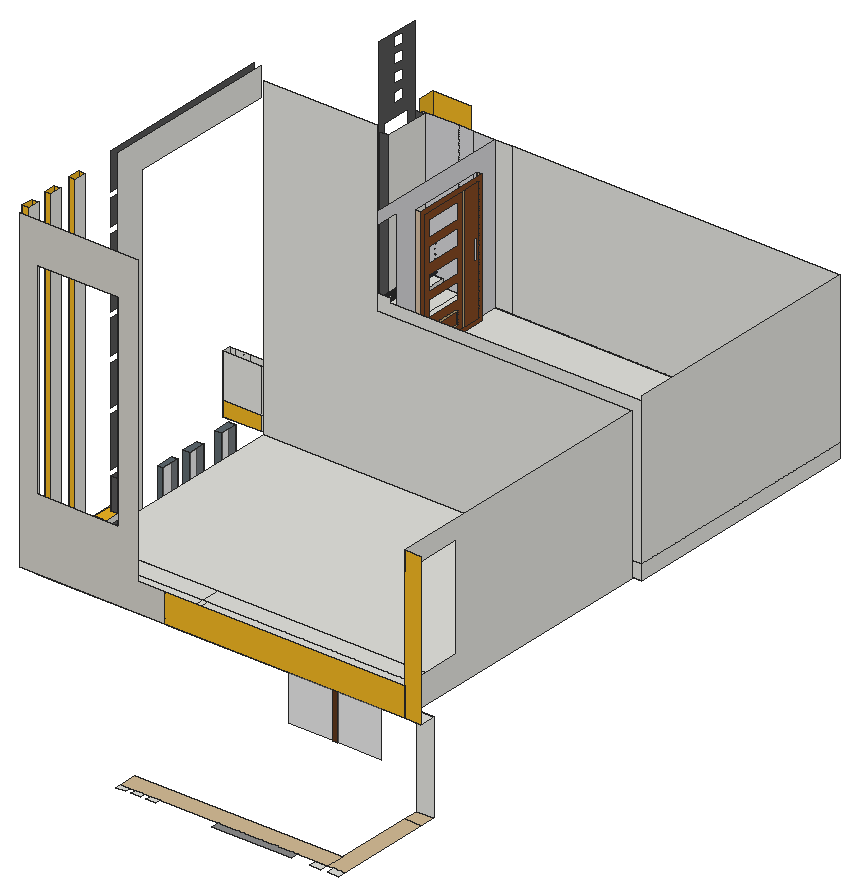
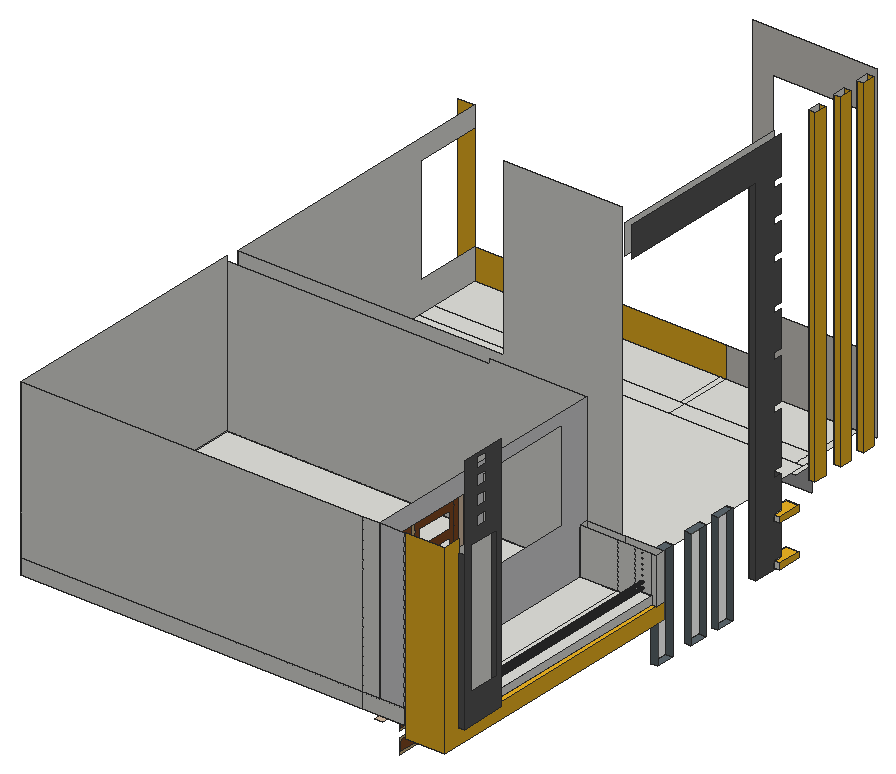
# SketchUp Ruby script. Lengths in inches.
U = 1.inch
M = Sketchup.active_model
def pt(a) = Geom::Point3d.new(a.map { |v| v * U })
def face(e, loops, mat)
  f = e.add_face(loops[0].map { |a| pt(a) })
  loops[1..].each { |l| e.add_face(l.map { |a| pt(a) }).erase! }
  f.material = f.back_material = mat if mat
  f
end
# faces: each face lists its corners as indices into pts; further lists are holes
def faces(e, pts, list, mat = nil) = list.each { |f| face(e, (f[0].is_a?(Array) ? f : [f]).map { |l| l.map { |i| pts[i] } }, mat) }
# xy, xz, yz: faces in a plane at the given z, y or x. An outline is a flat list of corners, or four numbers for a rectangle; further outlines are holes
def ring(l) = l.size == 4 ? [[l[0], l[1]], [l[2], l[1]], [l[2], l[3]], [l[0], l[3]]] : l.each_slice(2).to_a
def flat(e, list, mat, &to3) = list.each { |f| face(e, (f[0].is_a?(Array) ? f : [f]).map { |l| ring(l).map { |u, v| to3.(u, v) } }, mat) }
def xy(e, z, list, mat = nil) = flat(e, list, mat) { |x, y| [x, y, z] }
def xz(e, y, list, mat = nil) = flat(e, list, mat) { |x, z| [x, y, z] }
def yz(e, x, list, mat = nil) = flat(e, list, mat) { |y, z| [x, y, z] }
def lines(e, pts, list) = list.each { |a, b| e.add_line(pt(pts[a]), pt(pts[b])) }
# prism: a flat outline (further loops are holes) pulled along v
def prism(e, loops, v, mat = nil)
  f = face(e, loops, mat); d = Geom::Vector3d.new(v.map { |x| x * U })
  f.pushpull(f.normal.samedirection?(d) ? d.length : -d.length)
end
def box(e, o, s, mat = nil) = prism(e, [[o, [o[0] + s[0], o[1], o[2]], [o[0] + s[0], o[1] + s[1], o[2]], [o[0], o[1] + s[1], o[2]]]], [0, 0, s[2]], mat)
def at(x, y, z, deg = 0) = Geom::Transformation.translation(pt([x, y, z])) * Geom::Transformation.rotation(ORIGIN, Z_AXIS, deg.degrees)
def axes(o, x, y, z) = Geom::Transformation.new([*x, 0, *y, 0, *z, 0, *pt(o).to_a, 1])
def part(name) = M.definitions.add(name)
# library, detail: a bought-in or finely detailed component or shape, given as its bounding box
def library(name, o, s) = part(name).tap { |d| box(d.entities, o, s) }
def detail(e, o, s) = box(e.add_group.entities, o, s)
def put(e, d, t, mat = nil) = e.add_instance(d, t).tap { |i| i.material = mat if mat }
def group(e, t, mat = nil) = e.add_group.tap { |g| g.transformation = t; g.material = mat if mat }.entities
root = M.entities
M.materials.add("[0045_Goldenrod]").color = [239, 181, 35]
M.materials.add("[Blinds Vertical Pattern]").color = [212, 212, 214]
M.materials.add("[Color M04]").color = [142, 142, 142]
M.materials.add("[Color M06]").color = [86, 86, 86]
M.materials.add("[Color M07]").color = [58, 58, 58]
M.materials.add("[Fencing Picket Concave]").color = [160, 160, 160]
M.materials.add("[Formica Beige]").color = [211, 187, 149]
M.materials.add("[Formica Laminate Light]").color = [213, 189, 164]
M.materials.add("[Formica Speckled Grey]").color = [94, 105, 111]
M.materials.add("[Tile Travertine 2 inch]").color = [211, 208, 201]
M.materials.add("[Translucent Glass Gray]").color = [145, 145, 145]
M.materials["[Translucent Glass Gray]"].alpha = 0.5
M.materials.add("[Translucent Glass Gray]1").color = [128, 128, 128]
M.materials["[Translucent Glass Gray]1"].alpha = 0.5
M.materials.add("[Wood Cherry Original]").color = [130, 73, 35]
M.materials.add("[Wood Floor Light]").color = [204, 176, 127]
M.materials.add("[Wood Veneer 01]").color = [96, 56, 29]
xy(root,89.5625,[[499.38,0,512.5625,9.1875],[520.19,0,533.375,9.1875],[265.43,2.6875,276.6,9.1875],[283.37,2.6875,294.54,9.1875],[301.06,2.6875,312.23,9.1875]])
xy(root,89.5625,[[382.41,0,477.59,9.1875]],"[Color M04]")
xy(root,89.5625,[[265.43,9.1875,513.45,31.125],[513.45,9.1875,533.375,123.625],[513.45,123.625,533.375,142.4375]],"[Formica Beige]")
xy(root,101.04,[[53.375,329.87,59.9375,351.12],[53.375,367.37,61.125,388.62],[53.375,415.12,61.375,436.37]],"[Formica Speckled Grey]")
xy(root,134.2,[[45.3125,270.46,53.375,306.125]],"[Color M06]")
xy(root,136.59,[[38.625,253.03,38.625,280.03,45.3125,280.03,45.3125,270.46,53.375,270.46,53.375,253.03]],"[0045_Goldenrod]")
xy(root,143.41,[[38.625,253.03,53.375,253.03,53.375,270.46,45.3125,270.46,45.3125,280.03,38.625,280.03]],"[0045_Goldenrod]")
xy(root,160.59,[[116.75,663.47,125.57,751.59]],"[Formica Laminate Light]")
xy(root,164.17,[[106.94,539.02,116.75,631.05],[116.75,539.02,128.38,631.05]])
xy(root,167.75,[[311.03,171.21,433.4,181.59],[311.03,181.59,433.4,197.15]])
xy(root,174.66,[[106.94,528.53,116.75,641.54]])
xy(root,183.35,[[295.4375,171.21,449,181.59]])
xy(root,184.34,[[38.625,253.03,38.625,280.03,45.3125,280.03,45.3125,270.46,53.375,270.46,53.375,253.03]],"[0045_Goldenrod]")
xy(root,185.6875,[[53.375,483.625,116.75,779.875],[116.75,483.625,509.21,779.875]])
xy(root,185.6875,[[8.375,483.625,53.375,779.875],[8.375,779.875,18.625,797.6875]],"[0045_Goldenrod]")
xy(root,186,[[81.47,181.59,226.34,204.11]])
xy(root,191.16,[[38.625,253.03,53.375,253.03,53.375,270.46,45.3125,270.46,45.3125,280.03,38.625,280.03]],"[0045_Goldenrod]")
xy(root,198,[[73.3,123.625,81.47,181.59],[81.47,123.625,226.34,181.59],[226.34,123.625,231.56,181.59],[231.56,123.625,513.45,181.59],[513.45,123.625,533.375,142.4375],
  [73.3,181.59,81.47,204.11],[81.47,181.59,226.34,204.11],[226.34,181.59,513.45,204.11],[73.3,204.11,513.45,463.7]])
xy(root,198,[[45.75,136.75,53.375,151.32],[45.75,169.81,53.375,184.38],[45.75,206.12,53.375,220.7]],"[0045_Goldenrod]")
xy(root,203.25,[[8.375,483.625,97.02,493.85],[97.02,483.625,97.02,660.4,103.59,660.4,103.59,752.02,97.02,752.02,97.02,779.875,509.21,779.875,509.21,483.625],[14.37,493.85,33.87,779.875],[33.87,493.85,53.375,779.875],[53.375,493.85,97.02,493.85,97.02,660.4,103.59,660.4,103.59,752.02,97.02,752.02,97.02,779.875,53.375,779.875],
  [8.375,724.47,14.37,777.2],[8.375,777.2,14.37,779.875]])
xy(root,203.25,[[8.375,493.85,14.37,724.47]],"[0045_Goldenrod]")
xy(root,203.25,[[2.5625,724.47,8.375,777.2]],"[Color M06]")
xy(root,212.375,[[14.37,493.85,33.87,779.875]])
xy(root,216.42,[[53.375,329.87,59.9375,351.12],[53.375,367.37,61.125,388.62],[53.375,415.12,61.375,436.37]],"[Formica Speckled Grey]")
xz(root,123.625,[[226.34,198,513.45,232.59],[513.45,198,533.375,378]],"[0045_Goldenrod]")
xz(root,123.625,[[[53.375,198,226.34,198,226.34,232.59,194.63,232.59,194.63,577.3125,53.375,577.3125],[73.3,283.375,172.24,529.3125]]],"[Tile Travertine 2 inch]")
xz(root,136.75,[[45.75,198,53.375,577.3125]],"[0045_Goldenrod]")
xz(root,142.4375,[[513.45,89.5625,533.375,198]])
xz(root,151.32,[[45.75,198,53.375,577.3125]],"[0045_Goldenrod]")
xz(root,169.81,[[45.75,198,53.375,577.3125]],"[0045_Goldenrod]")
xz(root,181.59,[[81.47,156.98,226.34,186]],"[Fencing Picket Concave]")
xz(root,184.38,[[45.75,198,53.375,577.3125]],"[0045_Goldenrod]")
xz(root,197.15,[[316.66,90.2,368.6,162.125],[375.03,90.2,427.78,162.125]],"[Translucent Glass Gray]")
xz(root,197.15,[[368.6,90.2,375.03,162.125]],"[Wood Veneer 01]")
xz(root,206.12,[[45.75,198,53.375,577.3125]],"[0045_Goldenrod]")
xz(root,220.7,[[45.75,198,53.375,577.3125]],"[0045_Goldenrod]")
xz(root,253.03,[[38.625,136.59,53.375,143.41],[38.625,184.34,53.375,191.16]],"[0045_Goldenrod]")
xz(root,270.46,[[45.3125,136.59,53.375,143.41],[45.3125,184.34,53.375,191.16]])
xz(root,270.46,[[45.3125,134.2,53.375,136.59],[45.3125,143.41,53.375,184.34],[45.3125,191.16,53.375,228.72]],"[Color M06]")
xz(root,280.03,[[38.625,136.59,45.3125,143.41],[38.625,184.34,45.3125,191.16]])
xz(root,306.125,[[45.3125,134.2,53.375,543.2]],"[Color M06]")
xz(root,329.87,[[53.375,101.04,59.9375,216.42]],"[Formica Speckled Grey]")
xz(root,351.12,[[53.375,101.04,59.9375,216.42]],"[Formica Speckled Grey]")
xz(root,367.37,[[53.375,101.04,61.125,216.42]],"[Formica Speckled Grey]")
xz(root,388.62,[[53.375,101.04,61.125,216.42]],"[Formica Speckled Grey]")
xz(root,415.12,[[53.375,101.04,61.375,216.42]],"[Formica Speckled Grey]")
xz(root,436.37,[[53.375,101.04,61.375,216.42]],"[Formica Speckled Grey]")
xz(root,463.7,[[73.3,198,73.3,577.3125,208.03,577.3125,208.03,378,513.45,378,513.45,198]])
xz(root,483.625,[[53.375,185.6875,509.21,203.25],[8.375,203.25,53.375,255.625],[53.375,203.25,97.02,255.625],[97.02,203.25,97.02,383.375,208.03,383.375,208.03,378,509.21,378,509.21,203.25]])
xz(root,483.625,[[8.375,185.6875,53.375,203.25]],"[0045_Goldenrod]")
xz(root,493.85,[[8.375,203.25,14.37,255.625],[14.37,203.25,33.87,212.375],[33.87,203.25,53.375,255.625],[53.375,203.25,97.02,255.625],[[14.37,212.375,33.87,255.625],[25.42,214.97,25.79,215.02,26.14,215.16,26.4375,215.39,26.66,215.69,26.81,216.04,26.86,216.41,26.81,216.78,26.66,217.13,26.4375,217.43,26.14,217.65,25.79,217.8,25.42,217.85,25.05,217.8,24.7,217.65,24.4,217.43,24.17,217.13,24.03,216.78,23.98,216.41,24.03,216.04,24.17,215.69,24.4,215.39,24.7,215.16,25.05,215.02],[25.42,251.22,25.79,251.27,26.14,251.41,26.4375,251.64,26.66,251.94,26.81,252.29,26.86,252.66,26.81,253.03,26.66,253.38,26.4375,253.68,26.14,253.9,25.79,254.05,25.42,254.1,25.05,254.05,24.7,253.9,24.4,253.68,24.17,253.38,24.03,253.03,23.98,252.66,24.03,252.29,24.17,251.94,24.4,251.64,24.7,251.41,25.05,251.27],[25.42,221.16,25.79,221.21,26.14,221.35,26.4375,221.58,26.66,221.88,26.81,222.22,26.86,222.6,26.81,222.97,26.66,223.32,26.4375,223.61,26.14,223.84,25.79,223.99,25.42,224.03,25.05,223.99,24.7,223.84,24.4,223.61,24.17,223.32,24.03,222.97,23.98,222.6,24.03,222.22,24.17,221.88,24.4,221.58,24.7,221.35,25.05,221.21],[25.42,245.53,25.79,245.58,26.14,245.73,26.4375,245.96,26.66,246.25,26.81,246.6,26.86,246.97,26.81,247.34,26.66,247.69,26.4375,247.99,26.14,248.22,25.79,248.36,25.42,248.41,25.05,248.36,24.7,248.22,24.4,247.99,24.17,247.69,24.03,247.34,23.98,246.97,24.03,246.6,24.17,246.25,24.4,245.96,24.7,245.73,25.05,245.58],[25.42,228.28,25.79,228.33,26.14,228.48,26.4375,228.71,26.66,229,26.81,229.35,26.86,229.72,26.81,230.09,26.66,230.44,26.4375,230.74,26.14,230.97,25.79,231.11,25.42,231.16,25.05,231.11,24.7,230.97,24.4,230.74,24.17,230.44,24.03,230.09,23.98,229.72,24.03,229.35,24.17,229,24.4,228.71,24.7,228.48,25.05,228.33],[25.42,239.53,25.79,239.58,26.14,239.73,26.4375,239.96,26.66,240.25,26.81,240.6,26.86,240.97,26.81,241.34,26.66,241.69,26.4375,241.99,26.14,242.22,25.79,242.36,25.42,242.41,25.05,242.36,24.7,242.22,24.4,241.99,24.17,241.69,24.03,241.34,23.98,240.97,24.03,240.6,24.17,240.25,24.4,239.96,24.7,239.73,25.05,239.58],[25.42,233.97,25.79,234.02,26.14,234.16,26.4375,234.39,26.66,234.69,26.81,235.04,26.86,235.41,26.81,235.78,26.66,236.13,26.4375,236.43,26.14,236.65,25.79,236.8,25.42,236.85,25.05,236.8,24.7,236.65,24.4,236.43,24.17,236.13,24.03,235.78,23.98,235.41,24.03,235.04,24.17,234.69,24.4,234.39,24.7,234.16,25.05,234.02]],
  [25.42,214.97,25.79,215.02,26.14,215.16,26.4375,215.39,26.66,215.69,26.81,216.04,26.86,216.41,26.81,216.78,26.66,217.13,26.4375,217.43,26.14,217.65,25.79,217.8,25.42,217.85,25.05,217.8,24.7,217.65,24.4,217.43,24.17,217.13,24.03,216.78,23.98,216.41,24.03,216.04,24.17,215.69,24.4,215.39,24.7,215.16,25.05,215.02],[25.42,221.16,25.79,221.21,26.14,221.35,26.4375,221.58,26.66,221.88,26.81,222.22,26.86,222.6,26.81,222.97,26.66,223.32,26.4375,223.61,26.14,223.84,25.79,223.99,25.42,224.03,25.05,223.99,24.7,223.84,24.4,223.61,24.17,223.32,24.03,222.97,23.98,222.6,24.03,222.22,24.17,221.88,24.4,221.58,24.7,221.35,25.05,221.21]])
xz(root,660.4,[[97.02,203.25,103.59,360.75]],"[Formica Laminate Light]")
xz(root,724.47,[[2.5625,203.25,14.37,383.375]],"[Color M06]")
xz(root,752.02,[[97.02,203.25,103.59,360.75]],"[Formica Laminate Light]")
xz(root,777.2,[[2.5625,203.25,14.37,383.375]],"[Color M06]")
xz(root,779.875,[[70.21,185.6875,116.75,203.25],[116.75,185.6875,509.21,203.25],[14.37,203.25,33.87,212.375],[97.02,203.25,116.75,383.375],[116.75,203.25,509.21,383.375]])
xz(root,779.875,[[[8.375,203.25,14.37,203.25,14.37,212.375,33.87,212.375,33.87,203.25,53.375,203.25,53.375,383.375,8.375,383.375],[25.42,251.22,25.05,251.27,24.7,251.41,24.4,251.64,24.17,251.94,24.03,252.29,23.98,252.66,24.03,253.03,24.17,253.38,24.4,253.68,24.7,253.9,25.05,254.05,25.42,254.1,25.79,254.05,26.14,253.9,26.4375,253.68,26.66,253.38,26.81,253.03,26.86,252.66,26.81,252.29,26.66,251.94,26.4375,251.64,26.14,251.41,25.79,251.27],[25.42,214.97,25.05,215.02,24.7,215.16,24.4,215.39,24.17,215.69,24.03,216.04,23.98,216.41,24.03,216.78,24.17,217.13,24.4,217.43,24.7,217.65,25.05,217.8,25.42,217.85,25.79,217.8,26.14,217.65,26.4375,217.43,26.66,217.13,26.81,216.78,26.86,216.41,26.81,216.04,26.66,215.69,26.4375,215.39,26.14,215.16,25.79,215.02],[25.42,221.16,25.05,221.21,24.7,221.35,24.4,221.58,24.17,221.88,24.03,222.22,23.98,222.6,24.03,222.97,24.17,223.32,24.4,223.61,24.7,223.84,25.05,223.99,25.42,224.03,25.79,223.99,26.14,223.84,26.4375,223.61,26.66,223.32,26.81,222.97,26.86,222.6,26.81,222.22,26.66,221.88,26.4375,221.58,26.14,221.35,25.79,221.21],[25.42,228.28,25.05,228.33,24.7,228.48,24.4,228.71,24.17,229,24.03,229.35,23.98,229.72,24.03,230.09,24.17,230.44,24.4,230.74,24.7,230.97,25.05,231.11,25.42,231.16,25.79,231.11,26.14,230.97,26.4375,230.74,26.66,230.44,26.81,230.09,26.86,229.72,26.81,229.35,26.66,229,26.4375,228.71,26.14,228.48,25.79,228.33],[25.42,233.97,25.05,234.02,24.7,234.16,24.4,234.39,24.17,234.69,24.03,235.04,23.98,235.41,24.03,235.78,24.17,236.13,24.4,236.43,24.7,236.65,25.05,236.8,25.42,236.85,25.79,236.8,26.14,236.65,26.4375,236.43,26.66,236.13,26.81,235.78,26.86,235.41,26.81,235.04,26.66,234.69,26.4375,234.39,26.14,234.16,25.79,234.02],[25.42,239.53,25.05,239.58,24.7,239.73,24.4,239.96,24.17,240.25,24.03,240.6,23.98,240.97,24.03,241.34,24.17,241.69,24.4,241.99,24.7,242.22,25.05,242.36,25.42,242.41,25.79,242.36,26.14,242.22,26.4375,241.99,26.66,241.69,26.81,241.34,26.86,240.97,26.81,240.6,26.66,240.25,26.4375,239.96,26.14,239.73,25.79,239.58],[25.42,245.53,25.05,245.58,24.7,245.73,24.4,245.96,24.17,246.25,24.03,246.6,23.98,246.97,24.03,247.34,24.17,247.69,24.4,247.99,24.7,248.22,25.05,248.36,25.42,248.41,25.79,248.36,26.14,248.22,26.4375,247.99,26.66,247.69,26.81,247.34,26.86,246.97,26.81,246.6,26.66,246.25,26.4375,245.96,26.14,245.73,25.79,245.58]],[53.375,203.25,70.21,383.375],[70.21,203.25,97.02,383.375]],"[Blinds Vertical Pattern]")
xz(root,797.6875,[[8.375,185.6875,53.375,396.875]],"[0045_Goldenrod]")
yz(root,2.5625,[[[724.47,203.25,777.2,479.1875],[731.17,238.4,767.73,388.58],[745.75,463.32,759.0625,475.07],[745.75,403.69,759.0625,415.44],[745.75,444.94,759.0625,456.69],[745.75,424.57,759.0625,436.32]]],"[Color M06]")
yz(root,8.375,[[483.625,203.25,493.85,255.625]])
yz(root,8.375,[[483.625,185.6875,483.625,203.25,779.875,203.25,779.875,383.375,777.2,383.375,777.2,396.875,797.6875,396.875,797.6875,185.6875]],"[0045_Goldenrod]")
yz(root,14.37,[[493.85,203.25,724.47,212.375],[724.47,203.25,777.2,212.375],[777.2,203.25,779.875,212.375],[724.47,212.375,777.2,383.375]])
yz(root,33.87,[[493.85,203.25,779.875,212.375]])
yz(root,38.625,[[253.03,136.59,280.03,143.41],[253.03,184.34,280.03,191.16]],"[0045_Goldenrod]")
yz(root,45.3125,[[270.46,136.59,280.03,143.41],[270.46,184.34,280.03,191.16]])
yz(root,45.3125,[[270.46,134.2,270.46,136.59,280.03,136.59,280.03,143.41,270.46,143.41,270.46,184.34,280.03,184.34,280.03,191.16,270.46,191.16,270.46,228.72,280.03,228.72,280.03,235.53,270.46,235.53,270.46,295.16,280.03,295.16,280.03,301.97,270.46,301.97,270.46,350.16,280.03,350.16,280.03,356.97,270.46,356.97,270.46,397.66,280.03,397.66,280.03,404.47,270.46,404.47,270.46,449.66,280.03,449.66,280.03,456.47,270.46,456.47,270.46,488.34,280.03,488.34,280.03,495.16,270.46,495.16,270.46,526.41,280.03,526.41,280.03,533.22,270.46,533.22,270.46,577.3125,483.625,577.3125,483.625,543.2,306.125,543.2,306.125,134.2]],"[Color M06]")
yz(root,45.75,[[136.75,198,151.32,577.3125],[169.81,198,184.38,577.3125],[206.12,198,220.7,577.3125]],"[0045_Goldenrod]")
yz(root,53.375,[[270.46,134.2,306.125,134.2,306.125,543.2,483.625,543.2,483.625,577.3125,270.46,577.3125],[253.03,136.59,270.46,143.41],[253.03,184.34,270.46,191.16],[136.75,198,151.32,577.3125],[169.81,198,184.38,577.3125],
  [206.12,198,220.7,577.3125]])
yz(root,59.9375,[[329.87,101.04,351.12,216.42]],"[Translucent Glass Gray]1")
yz(root,61.125,[[367.37,101.04,388.62,216.42]],"[Translucent Glass Gray]1")
yz(root,61.375,[[415.12,101.04,436.37,216.42]],"[Translucent Glass Gray]1")
yz(root,97.02,[[483.625,203.25,493.85,255.625]])
yz(root,97.02,[[[493.85,203.25,493.85,255.625,483.625,255.625,483.625,383.375,779.875,383.375,779.875,203.25,752.02,203.25,752.02,360.75,660.4,360.75,660.4,203.25],[518.89,265.95,632.14,369.45]]],"[Blinds Vertical Pattern]")
yz(root,103.59,[[[660.4,203.25,752.02,360.75],[665.42,208.27,747,355.73]],[[665.42,208.27,722.24,355.73],[671.74,327.91,715.87,346.72],[671.74,299.91,715.87,318.72],[671.74,269.85,715.87,288.66],[671.74,242.22,715.87,261.03],[671.74,213.85,715.87,232.66]],[[726.22,208.27,747,355.73],[739.76,272.3,743.82,296.74]],[675.22,217.32,712.4,229.1875]],"[Wood Cherry Original]")
yz(root,103.59,[[722.24,208.27,726.22,355.73],[[671.74,213.85,715.87,232.66],[675.22,217.32,712.4,229.1875]]],"[Wood Floor Light]")
yz(root,125.57,[[677.42,110.5625,714.18,122.58],[677.42,134.5,714.18,146.51]],"[Wood Cherry Original]")
yz(root,125.57,[[[675.02,108.16,716.58,124.98],[677.42,110.5625,714.18,122.58]],[[675.02,132.1,716.58,148.91],[677.42,134.5,714.18,146.51]]],"[Wood Floor Light]")
yz(root,509.21,[[483.625,185.6875,779.875,203.25],[483.625,203.25,779.875,383.375]])
yz(root,513.45,[[123.625,198,463.7,198,463.7,378,123.625,378,123.625,354.51,200.74,354.51,200.74,232.59,123.625,232.59]])
p = [[25.05,493.85,215.02],[24.7,493.85,215.16],[24.7,779.875,215.16],[25.05,779.875,215.02],[25.42,493.85,214.97],[25.42,779.875,214.97],
  [25.79,493.85,215.02],[25.79,779.875,215.02],[26.14,493.85,215.16],[26.14,779.875,215.16],[24.4,493.85,215.39],[24.4,779.875,215.39],
  [26.4375,493.85,215.39],[26.4375,779.875,215.39],[24.17,493.85,215.69],[24.17,779.875,215.69],[26.66,493.85,215.69],[26.66,779.875,215.69],
  [24.03,493.85,216.04],[24.03,779.875,216.04],[26.81,493.85,216.04],[26.81,779.875,216.04],[23.98,493.85,216.41],[23.98,779.875,216.41],
  [26.86,493.85,216.41],[26.86,779.875,216.41],[24.03,493.85,216.78],[24.03,779.875,216.78],[26.81,493.85,216.78],[26.81,779.875,216.78],
  [24.17,493.85,217.13],[24.17,779.875,217.13],[26.66,493.85,217.13],[26.66,779.875,217.13],[24.4,493.85,217.43],[24.4,779.875,217.43],
  [26.4375,493.85,217.43],[26.4375,779.875,217.43],[24.7,493.85,217.65],[24.7,779.875,217.65],[26.14,493.85,217.65],[26.14,779.875,217.65],
  [25.05,493.85,217.8],[25.05,779.875,217.8],[25.79,493.85,217.8],[25.79,779.875,217.8],[25.42,493.85,217.85],[25.42,779.875,217.85],
  [25.05,493.85,221.21],[24.7,493.85,221.35],[24.7,779.875,221.35],[25.05,779.875,221.21],[25.42,493.85,221.16],[25.42,779.875,221.16],
  [25.79,493.85,221.21],[25.79,779.875,221.21],[26.14,493.85,221.35],[26.14,779.875,221.35],[24.4,493.85,221.58],[24.4,779.875,221.58],
  [26.4375,493.85,221.58],[26.4375,779.875,221.58],[24.17,493.85,221.88],[24.17,779.875,221.88],[26.66,493.85,221.88],[26.66,779.875,221.88],
  [24.03,493.85,222.22],[24.03,779.875,222.22],[26.81,493.85,222.22],[26.81,779.875,222.22],[23.98,493.85,222.6],[23.98,779.875,222.6],
  [26.86,493.85,222.6],[26.86,779.875,222.6],[24.03,493.85,222.97],[24.03,779.875,222.97],[26.81,493.85,222.97],[26.81,779.875,222.97],
  [24.17,493.85,223.32],[24.17,779.875,223.32],[26.66,493.85,223.32],[26.66,779.875,223.32],[24.4,493.85,223.61],[24.4,779.875,223.61],
  [26.4375,493.85,223.61],[26.4375,779.875,223.61],[24.7,493.85,223.84],[24.7,779.875,223.84],[26.14,493.85,223.84],[26.14,779.875,223.84],
  [25.05,493.85,223.99],[25.05,779.875,223.99],[25.79,493.85,223.99],[25.79,779.875,223.99],[25.42,493.85,224.03],[25.42,779.875,224.03]]
faces(root,p,[[0,1,2,3],[4,0,3,5],[6,4,5,7],[8,6,7,9],[1,10,11,2],[12,8,9,13],[10,14,15,11],[16,12,13,17],
  [14,18,19,15],[20,16,17,21],[18,22,23,19],[24,20,21,25],[22,26,27,23],[28,24,25,29],[26,30,31,27],[32,28,29,33],
  [30,34,35,31],[36,32,33,37],[34,38,39,35],[40,36,37,41],[38,42,43,39],[44,40,41,45],[42,46,47,43],[46,44,45,47],
  [48,49,50,51],[52,48,51,53],[54,52,53,55],[56,54,55,57],[49,58,59,50],[60,56,57,61],[58,62,63,59],[64,60,61,65],
  [62,66,67,63],[68,64,65,69],[66,70,71,67],[72,68,69,73],[70,74,75,71],[76,72,73,77],[74,78,79,75],[80,76,77,81],
  [78,82,83,79],[84,80,81,85],[82,86,87,83],[88,84,85,89],[86,90,91,87],[92,88,89,93],[90,94,95,91],[94,92,93,95]],"[Color M07]")
